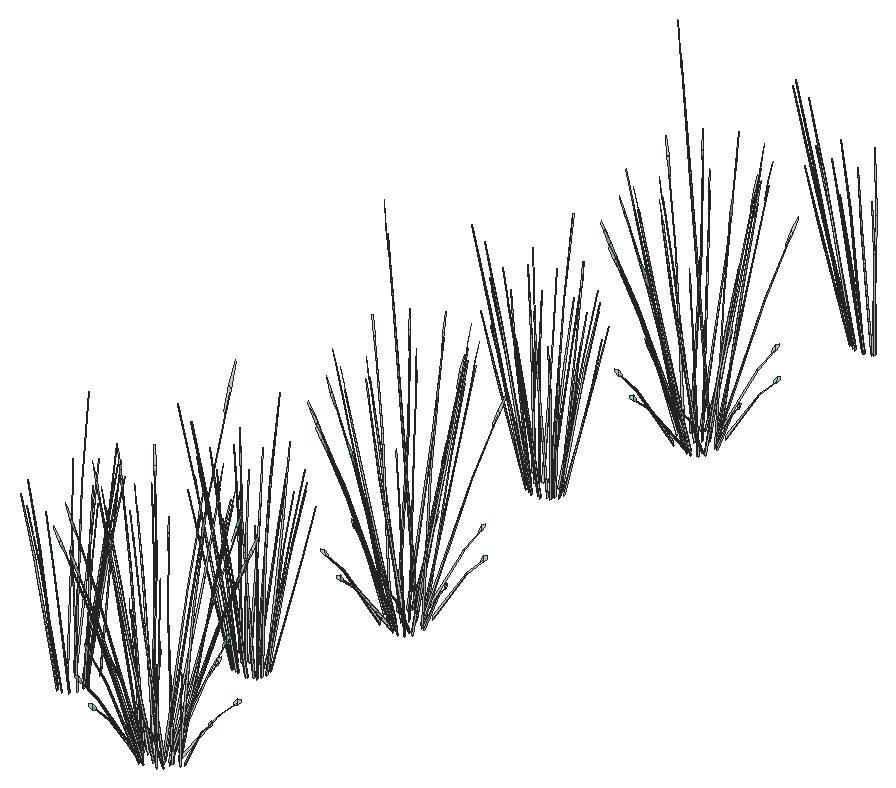
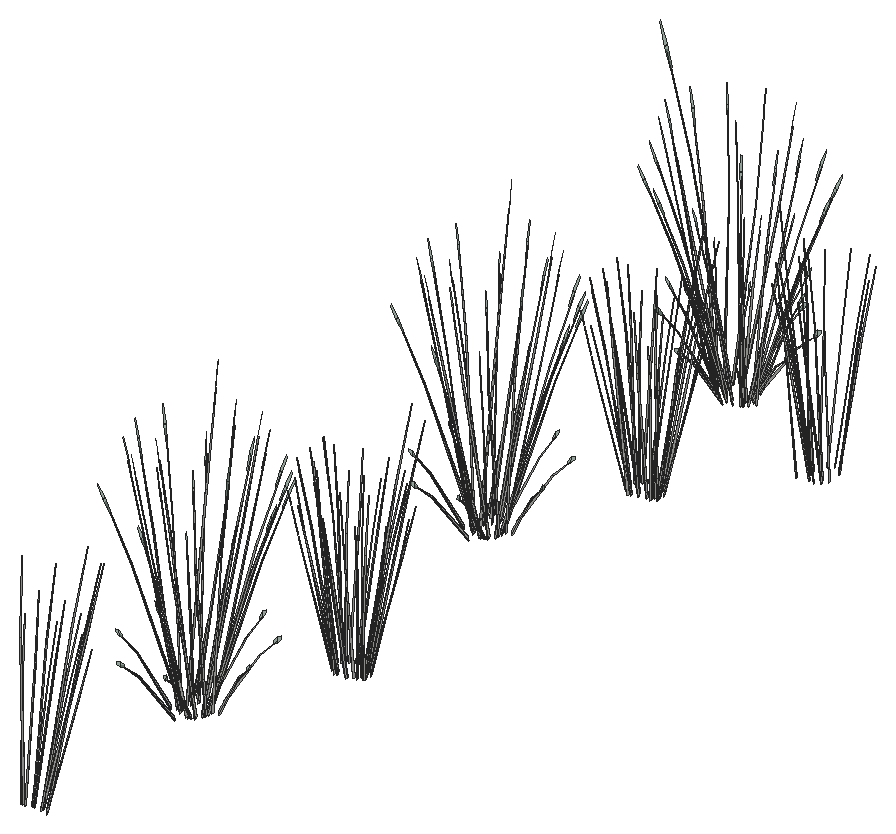
# SketchUp Ruby script. Lengths in inches.
U = 1.inch
M = Sketchup.active_model
def pt(a) = Geom::Point3d.new(a.map { |v| v * U })
def face(e, loops, mat)
  f = e.add_face(loops[0].map { |a| pt(a) })
  loops[1..].each { |l| e.add_face(l.map { |a| pt(a) }).erase! }
  f.material = f.back_material = mat if mat
  f
end
# faces: each face lists its corners as indices into pts; further lists are holes
def faces(e, pts, list, mat = nil) = list.each { |f| face(e, (f[0].is_a?(Array) ? f : [f]).map { |l| l.map { |i| pts[i] } }, mat) }
# xy, xz, yz: faces in a plane at the given z, y or x. An outline is a flat list of corners, or four numbers for a rectangle; further outlines are holes
def ring(l) = l.size == 4 ? [[l[0], l[1]], [l[2], l[1]], [l[2], l[3]], [l[0], l[3]]] : l.each_slice(2).to_a
def flat(e, list, mat, &to3) = list.each { |f| face(e, (f[0].is_a?(Array) ? f : [f]).map { |l| ring(l).map { |u, v| to3.(u, v) } }, mat) }
def xy(e, z, list, mat = nil) = flat(e, list, mat) { |x, y| [x, y, z] }
def xz(e, y, list, mat = nil) = flat(e, list, mat) { |x, z| [x, y, z] }
def yz(e, x, list, mat = nil) = flat(e, list, mat) { |y, z| [x, y, z] }
def lines(e, pts, list) = list.each { |a, b| e.add_line(pt(pts[a]), pt(pts[b])) }
# prism: a flat outline (further loops are holes) pulled along v
def prism(e, loops, v, mat = nil)
  f = face(e, loops, mat); d = Geom::Vector3d.new(v.map { |x| x * U })
  f.pushpull(f.normal.samedirection?(d) ? d.length : -d.length)
end
def box(e, o, s, mat = nil) = prism(e, [[o, [o[0] + s[0], o[1], o[2]], [o[0] + s[0], o[1] + s[1], o[2]], [o[0], o[1] + s[1], o[2]]]], [0, 0, s[2]], mat)
def at(x, y, z, deg = 0) = Geom::Transformation.translation(pt([x, y, z])) * Geom::Transformation.rotation(ORIGIN, Z_AXIS, deg.degrees)
def axes(o, x, y, z) = Geom::Transformation.new([*x, 0, *y, 0, *z, 0, *pt(o).to_a, 1])
def part(name) = M.definitions.add(name)
# library, detail: a bought-in or finely detailed component or shape, given as its bounding box
def library(name, o, s) = part(name).tap { |d| box(d.entities, o, s) }
def detail(e, o, s) = box(e.add_group.entities, o, s)
def put(e, d, t, mat = nil) = e.add_instance(d, t).tap { |i| i.material = mat if mat }
def group(e, t, mat = nil) = e.add_group.tap { |g| g.transformation = t; g.material = mat if mat }.entities
root = M.entities
M.materials.add("LightPink_Translucent").color = [175, 214, 192]
M.materials["LightPink_Translucent"].alpha = 0.75
c1 = part("blade")
p = [[2.15,0.21,22],[0,0.17,0],[0.09,0.45,0],[2.18,0.31,22],[2.29,0.31,22],[0.38,0.45,0],
  [2.48,0.24,33],[2.49,0.24,33],[2.48,0.22,33]]
faces(c1.entities,p,[[0,1,2,3],[4,5,2,3],[6,3,4,7],[8,0,3,6]])
c2 = part("blade with seeds\#1")
put(c2.entities,c1,at(0,0,0))
c3 = part("seeds")
p = [[0.3,-0.1,1.38],[-0.01,-0.03,1.59],[-0.01,-0.03,0.03],[0.14,-0.07,-0.07],[0.29,-0.03,3],[0.15,0.01,3.11]]
faces(c3.entities,p,[[0,1,2,3],[1,0,4,5]],"LightPink_Translucent")
c4 = part("blade with seeds")
put(c4.entities,c1,at(0,0,0))
put(c4.entities,c3,axes([2.4,0.25,30.99],[1.5799,-0.05474,1.17369],[-0.12525,1.92788,0.29478],[-0.07173,-0.02425,1.56792]))
put(root,c2,axes([472.2,241.91,140.86],[0.20062,0.33637,0.29052],[-0.22908,0.31842,-0.37506],[-0.11639,-0.04845,0.71765]))
put(root,c2,axes([471.92,243.9,140.86],[0.30692,-0.07678,0.29052],[0.08104,0.43892,-0.37506],[-0.08795,0.11789,0.71765]))
put(root,c2,axes([472.12,245.22,140.9],[-0.28121,-0.41055,0.44104],[0.29863,-0.35407,0.36366],[-0.05187,0.19262,0.91263]))
put(root,c2,axes([472.82,241.33,140.86],[0.05446,0.43273,0.29052],[-0.31131,0.11427,-0.37506],[-0.08362,-0.12401,0.71765]))
put(root,c2,axes([472.34,244.78,140.86],[0.23857,-0.28286,0.29052],[0.22584,0.32298,-0.37506],[-0.03436,0.1641,0.71765]))
put(root,c2,axes([473.57,241.26,140.86],[-0.1063,0.41315,0.29052],[-0.31012,-0.1205,-0.37506],[-0.02844,-0.16634,0.71765]))
put(root,c2,axes([473,245.24,140.86],[0.1063,-0.41315,0.29052],[0.31012,0.1205,-0.37506],[0.02844,0.16634,0.71765]))
put(root,c2,axes([474.24,241.72,140.86],[-0.23857,0.28286,0.29052],[-0.22584,-0.32298,-0.37506],[0.03436,-0.1641,0.71765]))
put(root,c2,axes([473.75,245.17,140.86],[-0.05446,-0.43273,0.29052],[0.31131,-0.11427,-0.37506],[0.08362,0.12401,0.71765]))
put(root,c2,axes([474.63,246.16,141.35],[0.10171,-0.43869,-0.05322],[0.31305,0.13494,-0.24131],[0.04753,0.07175,0.79594]))
put(root,c2,axes([474.65,242.6,140.86],[-0.30692,0.07678,0.29052],[-0.08104,-0.43892,-0.37506],[0.08795,-0.11789,0.71765]))
put(root,c2,axes([474.37,244.59,140.86],[-0.20062,-0.33637,0.29052],[0.22908,-0.31842,-0.37506],[0.11639,0.04845,0.71765]))
put(root,c2,axes([474.7,243.65,140.86],[-0.29303,-0.14987,0.29052],[0.08547,-0.43725,-0.37506],[0.11798,-0.04009,0.71765]))
put(root,c2,axes([475.74,243.06,141.35],[-0.2186,-0.34354,-0.05322],[0.23941,-0.31478,-0.24131],[0.06784,-0.02216,0.79594]))
put(root,c2,axes([474.94,243.65,140.87],[-0.09962,0.48986,0.43711],[-0.3275,-0.16751,0.36041],[0.12879,-0.02944,0.90448]))
put(root,c2,axes([483.76,257.39,140.6],[-0.18259,-0.25981,0.05275],[0.33295,-0.12717,0.41527],[-0.14677,0.02509,0.63322]))
put(root,c2,axes([483.76,307.375,140.6],[-0.18259,-0.25981,0.05275],[0.33295,-0.12717,0.41527],[-0.14677,0.02509,0.63322]))
put(root,c2,axes([484.15,256.6,140.9],[0.41055,-0.28121,0.44104],[0.35407,0.29863,0.36366],[-0.19262,-0.05187,0.91263]))
put(root,c2,axes([484.15,306.59,140.9],[0.41055,-0.28121,0.44104],[0.35407,0.29863,0.36366],[-0.19262,-0.05187,0.91263]))
put(root,c2,axes([483.81,258.28,140.6],[-0.34128,-0.16025,0.05275],[0.1987,-0.22821,0.41527],[-0.10942,0.07378,0.63322]))
put(root,c2,axes([483.81,308.27,140.6],[-0.34128,-0.16025,0.05275],[0.1987,-0.22821,0.41527],[-0.10942,0.07378,0.63322]))
put(root,c2,axes([484.13,257.48,140.86],[0.41315,0.1063,0.29052],[-0.1205,0.31012,-0.37506],[-0.16634,0.02844,0.71765]))
put(root,c2,axes([484.13,307.47,140.86],[0.41315,0.1063,0.29052],[-0.1205,0.31012,-0.37506],[-0.16634,0.02844,0.71765]))
put(root,c2,axes([484.34,256.6,140.6],[0.02503,-0.28975,0.05275],[0.378,0.00794,0.41527],[-0.1448,-0.03032,0.63322]))
put(root,c2,axes([484.34,306.59,140.6],[0.02503,-0.28975,0.05275],[0.378,0.00794,0.41527],[-0.1448,-0.03032,0.63322]))
put(root,c2,axes([484.6,256.82,140.86],[0.28286,0.23857,0.29052],[-0.32298,0.22584,-0.37506],[-0.1641,-0.03436,0.71765]))
put(root,c2,axes([484.6,306.8,140.86],[0.28286,0.23857,0.29052],[-0.32298,0.22584,-0.37506],[-0.1641,-0.03436,0.71765]))
put(root,c2,axes([483.22,259.11,141.35],[0.43869,0.10171,-0.05322],[-0.13494,0.31305,-0.24131],[-0.07175,0.04753,0.79594]))
put(root,c2,axes([483.22,309.1,141.35],[0.43869,0.10171,-0.05322],[-0.13494,0.31305,-0.24131],[-0.07175,0.04753,0.79594]))
put(root,c2,axes([484.2,258.23,140.86],[0.43273,-0.05446,0.29052],[0.11427,0.31131,-0.37506],[-0.12401,0.08362,0.71765]))
put(root,c2,axes([484.2,308.22,140.86],[0.43273,-0.05446,0.29052],[0.11427,0.31131,-0.37506],[-0.12401,0.08362,0.71765]))
put(root,c2,axes([484.48,259.03,140.6],[-0.40853,-0.01775,0.05275],[0.0112,-0.2681,0.41527],[-0.04275,0.1027,0.63322]))
put(root,c2,axes([484.48,309.02,140.6],[-0.40853,-0.01775,0.05275],[0.0112,-0.2681,0.41527],[-0.04275,0.1027,0.63322]))
put(root,c2,axes([485.47,256.4,140.86],[0.07678,0.30692,0.29052],[-0.43892,0.08104,-0.37506],[-0.11789,-0.08795,0.71765]))
put(root,c2,axes([485.47,306.39,140.86],[0.07678,0.30692,0.29052],[-0.43892,0.08104,-0.37506],[-0.11789,-0.08795,0.71765]))
put(root,c2,axes([485.28,256.04,140.9],[0.55379,-0.09794,0.44104],[0.09611,0.38419,0.36366],[-0.13024,-0.11323,0.91263]))
put(root,c2,axes([485.28,306.03,140.9],[0.55379,-0.09794,0.44104],[0.09611,0.38419,0.36366],[-0.13024,-0.11323,0.91263]))
put(root,c4,axes([488.86,235.6875,140.7],[0.19824,-0.01009,1.55952],[-0.13151,0.43714,0.1261],[-0.28251,-0.02704,0.66668]))
put(root,c2,axes([485.4,306.11,140.6],[0.22594,-0.24206,0.05275],[0.32175,0.14093,0.41527],[-0.10402,-0.07761,0.63322]))
put(root,c4,axes([488.94,236.46,140.7],[0.16583,-0.0942,1.55952],[0.13961,0.43527,0.1261],[-0.26034,0.09838,0.66668]))
put(root,c2,axes([484.79,258.85,140.86],[0.33637,-0.20062,0.29052],[0.31842,0.22908,-0.37506],[-0.04845,0.11639,0.71765]))
put(root,c2,axes([484.79,308.84,140.86],[0.33637,-0.20062,0.29052],[0.31842,0.22908,-0.37506],[-0.04845,0.11639,0.71765]))
put(root,c4,axes([488.4375,236.3,141.46],[-0.07805,0.05782,1.59199],[0.00664,0.42244,-0.25177],[-0.1789,0.05494,0.12768]))
put(root,c4,axes([489.24,234.99,140.7],[0.17753,0.07673,1.55952],[-0.36739,0.32188,0.1261],[-0.22898,-0.14521,0.66668]))
put(root,c4,axes([487.57,236.73,141.46],[0.061,0.01194,1.61419],[0.18869,0.39348,-0.15253],[-0.12486,0.10328,0.28566]))
put(root,c2,axes([486.52,256.35,140.86],[-0.14987,0.29303,0.29052],[-0.43725,-0.08547,-0.37506],[-0.04009,-0.11798,0.71765]))
put(root,c2,axes([486.52,306.34,140.86],[-0.14987,0.29303,0.29052],[-0.43725,-0.08547,-0.37506],[-0.04009,-0.11798,0.71765]))
put(root,c2,axes([485.72,259.42,140.87],[-0.48986,-0.09962,0.43711],[0.16751,-0.3275,0.36041],[0.02944,0.12879,0.90448]))
put(root,c2,axes([485.72,309.41,140.87],[-0.48986,-0.09962,0.43711],[0.16751,-0.3275,0.36041],[0.02944,0.12879,0.90448]))
put(root,c2,axes([485.59,309.43,140.6],[-0.36632,0.1295,0.05275],[-0.1793,-0.23615,0.41527],[0.03538,0.1041,0.63322]))
put(root,c4,axes([488.81,234.55,141.46],[0.03543,0.04444,1.61419],[-0.17081,0.3995,-0.15253],[-0.17299,0.00289,0.28566]))
put(root,c4,axes([489.2,234.28,141.46],[-0.10283,-0.00314,1.59199],[-0.32739,0.31434,-0.25177],[-0.17468,-0.06423,0.12768]))
put(root,c4,axes([488.9375,235.9,141.75],[0.24047,0.40325,-0.11066],[-0.4268,0.19816,-0.6142],[-0.17986,0.0532,0.93327]))
put(root,c4,axes([489.48,235.0625,141.75],[-0.02559,0.45289,-0.11066],[-0.48454,-0.01238,-0.6142],[-0.18661,-0.03146,0.93327]))
put(root,c4,axes([489.55,236.75,140.7],[0.11937,-0.13683,1.55952],[0.30141,0.36934,0.1261],[-0.20674,0.1682,0.66668]))
put(root,c2,axes([486.66,256.09,140.6],[0.36632,-0.1295,0.05275],[0.1793,0.23615,0.41527],[-0.03538,-0.1041,0.63322]))
put(root,c2,axes([486.66,306.07,140.6],[0.36632,-0.1295,0.05275],[0.1793,0.23615,0.41527],[-0.03538,-0.1041,0.63322]))
put(root,c4,axes([489.46,237.09,140.7],[0.08899,-0.15307,1.55952],[0.37333,0.31677,0.1261],[-0.16841,0.19743,0.66668]))
put(root,c2,axes([485.73,259.18,140.86],[0.14987,-0.29303,0.29052],[0.43725,0.08547,-0.37506],[0.04009,0.11798,0.71765]))
put(root,c2,axes([485.73,309.17,140.86],[0.14987,-0.29303,0.29052],[0.43725,0.08547,-0.37506],[0.04009,0.11798,0.71765]))
put(root,c4,axes([488.45,237.88,141.46],[-0.01188,0.08813,1.59199],[0.33715,0.30658,-0.25177],[-0.08826,0.14498,0.12768]))
put(root,c2,axes([486.32,260.22,141.35],[0.34354,-0.2186,-0.05322],[0.31478,0.23941,-0.24131],[0.02216,0.06784,0.79594]))
put(root,c2,axes([486.32,310.21,141.35],[0.34354,-0.2186,-0.05322],[0.31478,0.23941,-0.24131],[0.02216,0.06784,0.79594]))
put(root,c4,axes([488.96,236.86,141.75],[0.44211,0.24556,-0.11066],[-0.2547,0.35561,-0.6142],[-0.12491,0.12361,0.93327]))
put(root,c4,axes([490.4,274.87,141.46],[-0.07171,0.06058,1.59199],[-0.02817,0.48891,-0.25177],[-0.15815,0.04916,0.12768]))
put(root,c4,axes([490.4,324.86,141.46],[-0.07171,0.06058,1.59199],[-0.02817,0.48891,-0.25177],[-0.15815,0.04916,0.12768]))
put(root,c2,axes([487.46,256.68,140.86],[-0.33637,0.20062,0.29052],[-0.31842,-0.22908,-0.37506],[0.04845,-0.11639,0.71765]))
put(root,c2,axes([487.46,306.67,140.86],[-0.33637,0.20062,0.29052],[-0.31842,-0.22908,-0.37506],[0.04845,-0.11639,0.71765]))
put(root,c4,axes([491.96,274.75,140.7],[0.17092,-0.0117,1.55952],[-0.11339,0.50701,0.1261],[-0.24358,-0.03136,0.66668]))
put(root,c4,axes([491.96,324.74,140.7],[0.17092,-0.0117,1.55952],[-0.11339,0.50701,0.1261],[-0.24358,-0.03136,0.66668]))
put(root,c4,axes([490.3,233.39,141.46],[-0.00892,0.05338,1.61419],[-0.43976,0.19372,-0.15253],[-0.12941,-0.09903,0.28566]))
put(root,c4,axes([489.97,234.54,140.7],[0.10925,0.14298,1.55952],[-0.50484,0.12037,0.1261],[-0.1141,-0.22447,0.66668]))
put(root,c2,axes([486.85,259.41,140.6],[-0.22594,0.24206,0.05275],[-0.32175,-0.14093,0.41527],[0.10402,0.07761,0.63322]))
put(root,c2,axes([486.85,309.4,140.6],[-0.22594,0.24206,0.05275],[-0.32175,-0.14093,0.41527],[0.10402,0.07761,0.63322]))
put(root,c4,axes([492.04,275.65,140.7],[0.14298,-0.10925,1.55952],[0.12037,0.50484,0.1261],[-0.22447,0.1141,0.66668]))
put(root,c4,axes([492.04,325.63,140.7],[0.14298,-0.10925,1.55952],[0.12037,0.50484,0.1261],[-0.22447,0.1141,0.66668]))
put(root,c4,axes([491.23,274.98,141.75],[0.20734,0.4677,-0.11066],[-0.36799,0.22984,-0.6142],[-0.15507,0.06171,0.93327]))
put(root,c4,axes([491.23,324.97,141.75],[0.20734,0.4677,-0.11066],[-0.36799,0.22984,-0.6142],[-0.15507,0.06171,0.93327]))
put(root,c4,axes([491.49,272.93,141.46],[-0.08813,-0.01188,1.59199],[-0.30658,0.33715,-0.25177],[-0.14498,-0.08826,0.12768]))
put(root,c4,axes([491.49,322.92,141.46],[-0.08813,-0.01188,1.59199],[-0.30658,0.33715,-0.25177],[-0.14498,-0.08826,0.12768]))
put(root,c2,axes([486.78,259.13,140.86],[-0.07678,-0.30692,0.29052],[0.43892,-0.08104,-0.37506],[0.11789,0.08795,0.71765]))
put(root,c2,axes([486.78,309.12,140.86],[-0.07678,-0.30692,0.29052],[0.43892,-0.08104,-0.37506],[0.11789,0.08795,0.71765]))
put(root,c4,axes([492.29,273.94,140.7],[0.15307,0.08899,1.55952],[-0.31677,0.37333,0.1261],[-0.19743,-0.16841,0.66668]))
put(root,c4,axes([492.29,323.93,140.7],[0.15307,0.08899,1.55952],[-0.31677,0.37333,0.1261],[-0.19743,-0.16841,0.66668]))
put(root,c2,axes([487.77,256.5,140.6],[0.40853,0.01775,0.05275],[-0.0112,0.2681,0.41527],[0.04275,-0.1027,0.63322]))
put(root,c2,axes([487.77,306.49,140.6],[0.40853,0.01775,0.05275],[-0.0112,0.2681,0.41527],[0.04275,-0.1027,0.63322]))
put(root,c2,axes([491.6,352.49,140.99],[0.41055,-0.28121,0.44104],[0.35407,0.29863,0.36366],[-0.19262,-0.05187,0.91263]))
put(root,c4,axes([490.8,233.59,141.46],[-0.0731,-0.06244,1.59199],[-0.48785,0.03959,-0.25177],[-0.07786,-0.14934,0.12768]))
put(root,c2,axes([488.05,257.3,140.86],[-0.43273,0.05446,0.29052],[-0.11427,-0.31131,-0.37506],[0.12401,-0.08362,0.71765]))
put(root,c2,axes([488.05,307.29,140.86],[-0.43273,0.05446,0.29052],[-0.11427,-0.31131,-0.37506],[0.12401,-0.08362,0.71765]))
put(root,c2,axes([491.78,352.49,140.69],[0.02503,-0.28975,0.05275],[0.378,0.00794,0.41527],[-0.1448,-0.03032,0.63322]))
put(root,c2,axes([492.95,351.99,141.27],[-0.33178,0.3653,-0.11173],[-0.48049,-0.21045,-0.62013],[-0.16702,-0.10321,0.94228]))
put(root,c4,axes([492.625,274.03,140.7],[0.13683,0.11937,1.55952],[-0.36934,0.30141,0.1261],[-0.1682,-0.20674,0.66668]))
put(root,c4,axes([492.625,324.02,140.7],[0.13683,0.11937,1.55952],[-0.36934,0.30141,0.1261],[-0.1682,-0.20674,0.66668]))
put(root,c4,axes([491.54,234.56,141.75],[-0.4677,0.20734,-0.11066],[-0.22984,-0.36799,-0.6142],[-0.06171,-0.15507,0.93327]))
put(root,c4,axes([490.28,237.41,140.7],[-0.0117,-0.17092,1.55952],[0.50701,0.11339,0.1261],[-0.03136,0.24358,0.66668]))
put(root,c4,axes([491.24,276.09,141.75],[0.38119,0.2848,-0.11066],[-0.21961,0.41244,-0.6142],[-0.10769,0.14337,0.93327]))
put(root,c4,axes([491.24,326.08,141.75],[0.38119,0.2848,-0.11066],[-0.21961,0.41244,-0.6142],[-0.10769,0.14337,0.93327]))
put(root,c4,axes([492.51,273.4375,141.75],[-0.24556,0.44211,-0.11066],[-0.35561,-0.2547,-0.6142],[-0.12361,-0.12491,0.93327]))
put(root,c4,axes([492.51,323.42,141.75],[-0.24556,0.44211,-0.11066],[-0.35561,-0.2547,-0.6142],[-0.12361,-0.12491,0.93327]))
put(root,c4,axes([493.49,276.41,141.24],[0.23139,-0.41299,1.25837],[0.36026,0.43608,0.54295],[-0.21711,0.13325,1.21634]))
put(root,c4,axes([493.49,326.4,141.24],[0.23139,-0.41299,1.25837],[0.36026,0.43608,0.54295],[-0.21711,0.13325,1.21634]))
put(root,c4,axes([492.48,276.38,140.7],[0.07673,-0.17753,1.55952],[0.32188,0.36739,0.1261],[-0.14521,0.22898,0.66668]))
put(root,c4,axes([492.48,326.37,140.7],[0.07673,-0.17753,1.55952],[0.32188,0.36739,0.1261],[-0.14521,0.22898,0.66668]))
put(root,c2,axes([487.65,258.72,140.86],[-0.28286,-0.23857,0.29052],[0.32298,-0.22584,-0.37506],[0.1641,0.03436,0.71765]))
put(root,c2,axes([487.65,308.7,140.86],[-0.28286,-0.23857,0.29052],[0.32298,-0.22584,-0.37506],[0.1641,0.03436,0.71765]))
put(root,c2,axes([487.91,258.93,140.6],[-0.02503,0.28975,0.05275],[-0.378,-0.00794,0.41527],[0.1448,0.03032,0.63322]))
put(root,c2,axes([487.91,308.92,140.6],[-0.02503,0.28975,0.05275],[-0.378,-0.00794,0.41527],[0.1448,0.03032,0.63322]))
put(root,c2,axes([488.12,258.05,140.86],[-0.41315,-0.1063,0.29052],[0.1205,-0.31012,-0.37506],[0.16634,-0.02844,0.71765]))
put(root,c2,axes([488.12,308.03,140.86],[-0.41315,-0.1063,0.29052],[0.1205,-0.31012,-0.37506],[0.16634,-0.02844,0.71765]))
put(root,c2,axes([488.44,307.24,140.6],[0.34128,0.16025,0.05275],[-0.1987,0.22821,0.41527],[0.10942,-0.07378,0.63322]))
put(root,c2,axes([492.91,352.29,140.96],[0.07678,0.30692,0.29052],[-0.43892,0.08104,-0.37506],[-0.11789,-0.08795,0.71765]))
put(root,c2,axes([488.49,308.13,140.6],[0.18259,0.25981,0.05275],[-0.33295,0.12717,0.41527],[0.14677,-0.02509,0.63322]))
put(root,c4,axes([492.92,273.42,140.7],[0.0942,0.16583,1.55952],[-0.43527,0.13961,0.1261],[-0.09838,-0.26034,0.66668]))
put(root,c4,axes([492.92,323.41,140.7],[0.0942,0.16583,1.55952],[-0.43527,0.13961,0.1261],[-0.09838,-0.26034,0.66668]))
put(root,c4,axes([492.01,277.47,141.46],[0.00753,0.10253,1.59199],[0.34598,0.28122,-0.25177],[-0.04567,0.18237,0.12768]))
put(root,c4,axes([492.01,327.45,141.46],[0.00753,0.10253,1.59199],[0.34598,0.28122,-0.25177],[-0.04567,0.18237,0.12768]))
put(root,c2,axes([492.72,351.93,140.99],[0.55379,-0.09794,0.44104],[0.09611,0.38419,0.36366],[-0.13024,-0.11323,0.91263]))
put(root,c4,axes([490.39,238.97,141.46],[0.06058,0.07171,1.59199],[0.48891,0.02817,-0.25177],[0.04916,0.15815,0.12768]))
put(root,c2,axes([492.84,352.02,140.69],[0.22594,-0.24206,0.05275],[0.32175,0.14093,0.41527],[-0.10402,-0.07761,0.63322]))
put(root,c4,axes([491.73,277.04,141.75],[0.45289,0.02559,-0.11066],[-0.01238,0.48454,-0.6142],[-0.03146,0.18661,0.93327]))
put(root,c4,axes([491.73,327.03,141.75],[0.45289,0.02559,-0.11066],[-0.01238,0.48454,-0.6142],[-0.03146,0.18661,0.93327]))
put(root,c4,axes([493.47,273.42,141.75],[-0.40325,0.24047,-0.11066],[-0.19816,-0.4268,-0.6142],[-0.0532,-0.17986,0.93327]))
put(root,c4,axes([493.47,323.41,141.75],[-0.40325,0.24047,-0.11066],[-0.19816,-0.4268,-0.6142],[-0.0532,-0.17986,0.93327]))
put(root,c4,axes([493.07,272.92,141.46],[-0.05782,-0.07805,1.59199],[-0.42244,0.00664,-0.25177],[-0.05494,-0.1789,0.12768]))
put(root,c4,axes([493.07,322.9,141.46],[-0.05782,-0.07805,1.59199],[-0.42244,0.00664,-0.25177],[-0.05494,-0.1789,0.12768]))
put(root,c4,axes([490.5,238.15,141.75],[0.4677,-0.20734,-0.11066],[0.22984,0.36799,-0.6142],[0.06171,0.15507,0.93327]))
put(root,c4,axes([492.52,235.02,141.75],[-0.52527,-0.02206,-0.11066],[0.01436,-0.41777,-0.6142],[0.03649,-0.1609,0.93327]))
put(root,c4,axes([493.18,276.75,140.7],[-0.01009,-0.19824,1.55952],[0.43714,0.13151,0.1261],[-0.02704,0.28251,0.66668]))
put(root,c4,axes([493.18,326.74,140.7],[-0.01009,-0.19824,1.55952],[0.43714,0.13151,0.1261],[-0.02704,0.28251,0.66668]))
put(root,c2,axes([493.96,352.25,140.96],[-0.14987,0.29303,0.29052],[-0.43725,-0.08547,-0.37506],[-0.04009,-0.11798,0.71765]))
put(root,c4,axes([491.17,237.34,140.7],[-0.10925,-0.14298,1.55952],[0.50484,-0.12037,0.1261],[0.1141,0.22447,0.66668]))
put(root,c4,axes([491.93,235.88,141.24],[-0.41299,-0.23139,1.25837],[0.43608,-0.36026,0.54295],[0.13325,0.21711,1.21634]))
put(root,c4,axes([491.24,238.45,141.46],[0.00141,-0.05392,1.61419],[0.40958,-0.23787,-0.15253],[0.14227,0.0849,0.28566]))
put(root,c4,axes([492.99,234.36,141.46],[-0.00461,-0.08863,1.59199],[-0.38966,-0.25616,-0.25177],[0.06024,-0.15528,0.12768]))
put(root,c2,axes([494.1,351.98,140.69],[0.36632,-0.1295,0.05275],[0.1793,0.23615,0.41527],[-0.03538,-0.1041,0.63322]))
put(root,c2,axes([493.97,352.01,140.7],[0.48986,0.09962,0.39379],[-0.16751,0.3275,0.3247],[-0.02944,-0.12879,0.81485]))
put(root,c4,axes([493.6875,273.34,140.7],[0.01009,0.19824,1.55952],[-0.43714,-0.13151,0.1261],[0.02704,-0.28251,0.66668]))
put(root,c4,axes([493.6875,323.33,140.7],[0.01009,0.19824,1.55952],[-0.43714,-0.13151,0.1261],[0.02704,-0.28251,0.66668]))
put(root,c4,axes([492.57,277.58,141.75],[0.40325,-0.24047,-0.11066],[0.19816,0.4268,-0.6142],[0.0532,0.17986,0.93327]))
put(root,c4,axes([492.57,327.57,141.75],[0.40325,-0.24047,-0.11066],[0.19816,0.4268,-0.6142],[0.0532,0.17986,0.93327]))
put(root,c4,axes([494.3125,273.96,141.75],[-0.45289,-0.02559,-0.11066],[0.01238,-0.48454,-0.6142],[0.03146,-0.18661,0.93327]))
put(root,c4,axes([494.3125,323.95,141.75],[-0.45289,-0.02559,-0.11066],[0.01238,-0.48454,-0.6142],[0.03146,-0.18661,0.93327]))
put(root,c4,axes([491.67,234.79,140.7],[-0.08899,0.15307,1.55952],[-0.37333,-0.31677,0.1261],[0.16841,-0.19743,0.66668]))
put(root,c4,axes([491.61,238.13,141.75],[0.2848,-0.38119,-0.11066],[0.41244,0.21961,-0.6142],[0.14337,0.10769,0.93327]))
put(root,c4,axes([493.09,235.84,141.75],[-0.44211,-0.24556,-0.11066],[0.2547,-0.35561,-0.6142],[0.12491,-0.12361,0.93327]))
put(root,c4,axes([493.2,278.89,141.46],[0.06783,0.06632,1.59199],[0.4161,-0.08489,-0.25177],[0.07889,0.16641,0.12768]))
put(root,c4,axes([493.2,328.88,141.46],[0.06783,0.06632,1.59199],[0.4161,-0.08489,-0.25177],[0.07889,0.16641,0.12768]))
put(root,c2,axes([494.91,352.58,140.96],[-0.33637,0.20062,0.29052],[-0.31842,-0.22908,-0.37506],[0.04845,-0.11639,0.71765]))
put(root,c4,axes([491.9,236.89,140.7],[-0.17753,-0.07673,1.55952],[0.36739,-0.32188,0.1261],[0.22898,0.14521,0.66668]))
put(root,c4,axes([494.18,235.74,141.46],[-0.06243,-0.00338,1.61419],[-0.25923,-0.3624,-0.15253],[0.1041,-0.11916,0.28566]))
put(root,c4,axes([492.56,237.64,141.75],[0.02559,-0.45289,-0.11066],[0.48454,0.01238,-0.6142],[0.18661,0.03146,0.93327]))
put(root,c4,axes([493.11,236.8,141.75],[-0.24047,-0.40325,-0.11066],[0.4268,-0.19816,-0.6142],[0.17986,-0.0532,0.93327]))
put(root,c4,axes([493.53,277.57,141.75],[0.24556,-0.44211,-0.11066],[0.35561,0.2547,-0.6142],[0.12361,0.12491,0.93327]))
put(root,c4,axes([493.53,327.55,141.75],[0.24556,-0.44211,-0.11066],[0.35561,0.2547,-0.6142],[0.12361,0.12491,0.93327]))
put(root,c4,axes([495.1,273.68,141.46],[0.00314,-0.10283,1.59199],[-0.31434,-0.32739,-0.25177],[0.06423,-0.17468,0.12768]))
put(root,c4,axes([495.1,323.67,141.46],[0.00314,-0.10283,1.59199],[-0.31434,-0.32739,-0.25177],[0.06423,-0.17468,0.12768]))
put(root,c2,axes([495.21,352.39,140.69],[0.40853,0.01775,0.05275],[-0.0112,0.2681,0.41527],[0.04275,-0.1027,0.63322]))
put(root,c2,axes([495.08,352.37,140.7],[0.354,0.25999,0.39379],[-0.37594,0.22422,0.3247],[0.0653,-0.12198,0.81485]))
put(root,c4,axes([492.99,237.37,141.46],[0.10253,-0.00753,1.59199],[0.28122,-0.34598,-0.25177],[0.18237,0.04567,0.12768]))
put(root,c4,axes([494.39,273.72,140.7],[-0.07673,0.17753,1.55952],[-0.32188,-0.36739,0.1261],[0.14521,-0.22898,0.66668]))
put(root,c4,axes([494.39,323.7,140.7],[-0.07673,0.17753,1.55952],[-0.32188,-0.36739,0.1261],[0.14521,-0.22898,0.66668]))
put(root,c4,axes([492.27,236.19,140.7],[-0.19824,0.01009,1.55952],[0.13151,-0.43714,0.1261],[0.28251,0.02704,0.66668]))
put(root,c4,axes([494.35,276.99,141.75],[0.02206,-0.52527,-0.11066],[0.41777,0.01436,-0.6142],[0.1609,0.03649,0.93327]))
put(root,c4,axes([494.35,326.98,141.75],[0.02206,-0.52527,-0.11066],[0.41777,0.01436,-0.6142],[0.1609,0.03649,0.93327]))
put(root,c4,axes([494.82,276.02,141.75],[-0.20734,-0.4677,-0.11066],[0.36799,-0.22984,-0.6142],[0.15507,-0.06171,0.93327]))
put(root,c4,axes([494.82,326.01,141.75],[-0.20734,-0.4677,-0.11066],[0.36799,-0.22984,-0.6142],[0.15507,-0.06171,0.93327]))
put(root,c4,axes([494.41,236.17,141.46],[0.06632,-0.06783,1.59199],[-0.08489,-0.4161,-0.25177],[0.16641,-0.07889,0.12768]))
put(root,c4,axes([494.58,276.15,140.7],[-0.15307,-0.08899,1.55952],[0.31677,-0.37333,0.1261],[0.19743,0.16841,0.66668]))
put(root,c4,axes([494.58,326.14,140.7],[-0.15307,-0.08899,1.55952],[0.31677,-0.37333,0.1261],[0.19743,0.16841,0.66668]))
put(root,c4,axes([495.02,277.47,141.46],[0.08863,-0.00461,1.59199],[0.25616,-0.38966,-0.25177],[0.15528,0.06024,0.12768]))
put(root,c4,axes([495.02,327.46,141.46],[0.08863,-0.00461,1.59199],[0.25616,-0.38966,-0.25177],[0.15528,0.06024,0.12768]))
put(root,c4,axes([495.78,275.28,141.46],[0.06244,-0.0731,1.59199],[-0.03959,-0.48785,-0.25177],[0.14934,-0.07786,0.12768]))
put(root,c4,axes([495.78,325.27,141.46],[0.06244,-0.0731,1.59199],[-0.03959,-0.48785,-0.25177],[0.14934,-0.07786,0.12768]))
put(root,c4,axes([494.83,274.45,140.7],[-0.14298,0.10925,1.55952],[-0.12037,-0.50484,0.1261],[0.22447,-0.1141,0.66668]))
put(root,c4,axes([494.83,324.43,140.7],[-0.14298,0.10925,1.55952],[-0.12037,-0.50484,0.1261],[0.22447,-0.1141,0.66668]))
